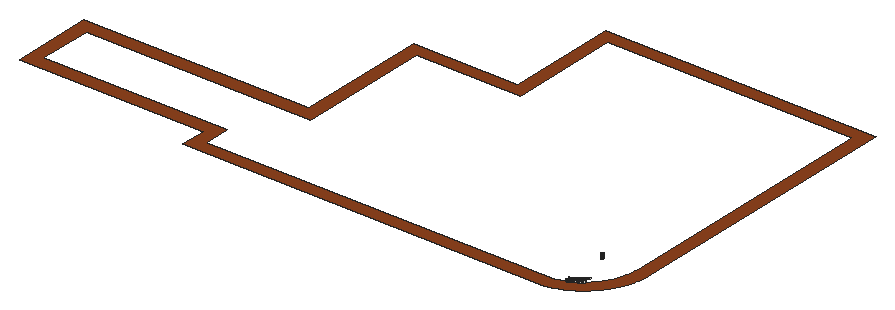
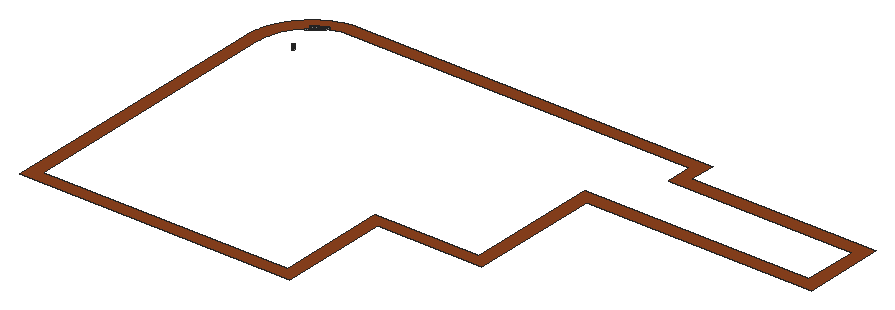
# SketchUp Ruby script. Lengths in inches.
U = 1.inch
M = Sketchup.active_model
def pt(a) = Geom::Point3d.new(a.map { |v| v * U })
def face(e, loops, mat)
  f = e.add_face(loops[0].map { |a| pt(a) })
  loops[1..].each { |l| e.add_face(l.map { |a| pt(a) }).erase! }
  f.material = f.back_material = mat if mat
  f
end
# faces: each face lists its corners as indices into pts; further lists are holes
def faces(e, pts, list, mat = nil) = list.each { |f| face(e, (f[0].is_a?(Array) ? f : [f]).map { |l| l.map { |i| pts[i] } }, mat) }
# xy, xz, yz: faces in a plane at the given z, y or x. An outline is a flat list of corners, or four numbers for a rectangle; further outlines are holes
def ring(l) = l.size == 4 ? [[l[0], l[1]], [l[2], l[1]], [l[2], l[3]], [l[0], l[3]]] : l.each_slice(2).to_a
def flat(e, list, mat, &to3) = list.each { |f| face(e, (f[0].is_a?(Array) ? f : [f]).map { |l| ring(l).map { |u, v| to3.(u, v) } }, mat) }
def xy(e, z, list, mat = nil) = flat(e, list, mat) { |x, y| [x, y, z] }
def xz(e, y, list, mat = nil) = flat(e, list, mat) { |x, z| [x, y, z] }
def yz(e, x, list, mat = nil) = flat(e, list, mat) { |y, z| [x, y, z] }
def lines(e, pts, list) = list.each { |a, b| e.add_line(pt(pts[a]), pt(pts[b])) }
# prism: a flat outline (further loops are holes) pulled along v
def prism(e, loops, v, mat = nil)
  f = face(e, loops, mat); d = Geom::Vector3d.new(v.map { |x| x * U })
  f.pushpull(f.normal.samedirection?(d) ? d.length : -d.length)
end
def box(e, o, s, mat = nil) = prism(e, [[o, [o[0] + s[0], o[1], o[2]], [o[0] + s[0], o[1] + s[1], o[2]], [o[0], o[1] + s[1], o[2]]]], [0, 0, s[2]], mat)
def at(x, y, z, deg = 0) = Geom::Transformation.translation(pt([x, y, z])) * Geom::Transformation.rotation(ORIGIN, Z_AXIS, deg.degrees)
def axes(o, x, y, z) = Geom::Transformation.new([*x, 0, *y, 0, *z, 0, *pt(o).to_a, 1])
def part(name) = M.definitions.add(name)
# library, detail: a bought-in or finely detailed component or shape, given as its bounding box
def library(name, o, s) = part(name).tap { |d| box(d.entities, o, s) }
def detail(e, o, s) = box(e.add_group.entities, o, s)
def put(e, d, t, mat = nil) = e.add_instance(d, t).tap { |i| i.material = mat if mat }
def group(e, t, mat = nil) = e.add_group.tap { |g| g.transformation = t; g.material = mat if mat }.entities
root = M.entities
M.materials.add("[Wood Fence]").color = [142, 67, 30]
xy(root,107.5,[[[126.5,152,126.5,166,26,166,26,210,149,210,149,282,206,282,206,342,354,342,354,186.72,353.99,186.41,353.98,186.09,353.96,185.77,353.95,185.45,353.93,185.13,353.9,184.8125,353.88,184.5,353.79,183.54,353.75,183.23,353.67,182.59,353.625,182.28,353.58,181.96,353.53,181.65,353.47,181.33,353.42,181.02,353.36,180.71,353.3,180.39,352.95,178.84,352.79,178.22,352.7,177.91,352.62,177.6,352.53,177.3,352.4375,176.99,352.34,176.6875,352.25,176.38,352.15,176.08,352.04,175.78,351.9375,175.48,351.83,175.18,351.61,174.58,351.49,174.28,351.37,173.99,351.25,173.69,351.13,173.4,351,173.11,350.875,172.8125,350.74,172.52,350.61,172.23,350.47,171.95,350.19,171.37,350.05,171.09,349.9,170.81,349.75,170.52,349.45,169.96,349.29,169.6875,349.13,169.41,348.97,169.13,348.8,168.86,348.64,168.59,348.3,168.05,348.125,167.78,347.95,167.52,347.77,167.25,347.41,166.73,346.84,165.95,346.65,165.7,346.46,165.44,346.26,165.19,346.0625,164.94,345.86,164.7,345.66,164.45,345.45,164.21,345.25,163.96,345.04,163.72,344.83,163.49,344.61,163.25,344.4,163.01,343.74,162.32,343.29,161.87,342.6,161.21,342.36,160.99,342.125,160.77,341.89,160.5625,341.65,160.35,341.41,160.14,341.16,159.9375,340.92,159.73,340.17,159.13,339.92,158.9375,339.67,158.75,339.41,158.55,339.15,158.37,338.9,158.18,338.64,158,338.375,157.8125,338.11,157.63,337.84,157.46,337.58,157.28,336.77,156.77,336.49,156.61,336.22,156.45,335.94,156.29,335.67,156.13,335.39,155.97,334.83,155.67,334.54,155.52,334.26,155.38,333.98,155.23,333.6875,155.09,333.4,154.96,333.11,154.82,332.82,154.6875,332.53,154.56,332.24,154.43,331.95,154.31,331.65,154.18,331.36,154.06,331.06,153.95,330.76,153.83,330.16,153.61,329.86,153.51,329.56,153.4,329.26,153.3,328.95,153.2,328.65,153.11,328.35,153.01,328.04,152.92,327.73,152.84,327.43,152.75,326.5,152.51,326.1875,152.44,325.88,152.37,325.57,152.3,325.25,152.23,324.63,152.11,324.3125,152.05,324,152],[133.5,159,323.38,159,323.59,159.04,323.84,159.09,324.1,159.14,325.1,159.38,325.34,159.44,326.09,159.65,326.33,159.72,326.58,159.79,326.83,159.87,327.07,159.95,327.3125,160.03,327.56,160.12,327.8,160.2,328.52,160.47,328.76,160.57,329,160.66,329.23,160.76,329.71,160.96,329.94,161.07,330.17,161.17,330.41,161.28,330.64,161.39,330.87,161.51,331.1,161.62,331.56,161.86,331.78,161.98,332.01,162.1,332.23,162.23,332.46,162.35,332.9,162.61,333.12,162.75,333.34,162.88,333.55,163.02,333.99,163.3,334.2,163.44,334.41,163.59,334.625,163.73,334.83,163.88,335.25,164.18,335.46,164.34,335.66,164.49,335.86,164.65,336.0625,164.81,336.26,164.97,336.46,165.13,336.66,165.3,336.86,165.46,337.24,165.8,337.4375,165.97,337.625,166.14,337.8125,166.32,338,166.49,338.1875,166.67,338.37,166.85,338.55,167.03,338.73,167.22,338.91,167.4,339.09,167.59,339.26,167.77,339.4375,167.96,339.61,168.15,339.78,168.35,339.95,168.54,340.12,168.74,340.28,168.93,340.45,169.13,340.93,169.73,341.08,169.9375,341.24,170.14,341.84,170.98,341.98,171.1875,342.125,171.4,342.27,171.61,342.55,172.05,342.68,172.27,342.82,172.48,342.95,172.7,343.08,172.93,343.21,173.15,343.33,173.37,343.46,173.6,343.58,173.82,343.82,174.28,343.93,174.51,344.05,174.74,344.27,175.2,344.375,175.43,344.48,175.67,344.59,175.9,344.6875,176.14,344.79,176.375,344.88,176.61,344.98,176.85,345.25,177.57,345.34,177.82,345.42,178.06,345.51,178.3,345.59,178.55,345.67,178.79,345.74,179.04,345.82,179.28,345.96,179.78,346.02,180.02,346.09,180.27,346.33,181.27,346.43,181.77,346.48,182.03,346.58,182.53,346.62,182.79,346.7,183.29,346.73,183.55,346.77,183.8,346.8,184.06,346.83,184.3125,346.86,184.57,346.88,184.82,346.92,185.34,346.94,185.59,346.96,185.85,346.97,186.1,346.99,186.62,347,186.875,347,335,213,335,213,275,156,275,156,203,33,203,33,173,133.5,173]]],"[Wood Fence]")
p = [[329.47,160.86,107.5],[329.23,160.76,107.5],[329.23,160.76,108.5],[329.47,160.86,108.5],[329.71,160.96,107.5],[329.71,160.96,108.5],
  [329.94,161.07,107.5],[329.94,161.07,108.5],[330.17,161.17,107.5],[330.17,161.17,108.5],[330.41,161.28,107.5],[330.41,161.28,108.5],
  [330.64,161.39,107.5],[330.64,161.39,108.5],[330.87,161.51,107.5],[330.87,161.51,108.5],[331.1,161.62,107.5],[331.1,161.62,108.5],
  [331.33,161.74,107.5],[331.33,161.74,108.5],[331.56,161.86,107.5],[331.56,161.86,108.5],[331.78,161.98,107.5],[331.78,161.98,108.5],
  [332.01,162.1,107.5],[332.01,162.1,108.5],[332.23,162.23,107.5],[332.23,162.23,108.5],[332.46,162.35,107.5],[332.46,162.35,108.5],
  [332.68,162.48,107.5],[332.68,162.48,108.5],[332.9,162.61,107.5],[332.9,162.61,108.5],[333.12,162.75,107.5],[333.12,162.75,108.5],
  [333.34,162.88,107.5],[333.34,162.88,108.5],[333.55,163.02,107.5],[333.55,163.02,108.5],[333.77,163.16,107.5],[333.77,163.16,108.5],
  [333.99,163.3,107.5],[333.99,163.3,108.5],[334.2,163.44,107.5],[334.2,163.44,108.5],[334.41,163.59,107.5],[334.41,163.59,108.5],
  [334.625,163.73,107.5],[334.625,163.73,108.5],[334.83,163.88,107.5],[334.83,163.88,108.5],[335.04,164.03,107.5],[335.04,164.03,108.5],
  [335.25,164.18,107.5],[335.25,164.18,108.5],[335.46,164.34,107.5],[335.46,164.34,108.5],[335.66,164.49,107.5],[335.66,164.49,108.5],
  [335.86,164.65,107.5],[335.86,164.65,108.5],[336.0625,164.81,107.5],[336.0625,164.81,108.5],[336.26,164.97,107.5],[336.26,164.97,108.5],
  [336.46,165.13,107.5],[336.46,165.13,108.5],[336.66,165.3,107.5],[336.66,165.3,108.5],[329.34,162.99,108],[329.55,163.09,108],
  [329.55,163.09,108.5],[329.34,162.99,108.5],[329.77,163.19,108],[329.77,163.19,108.5],[329.98,163.3,108],[329.98,163.3,108.5],
  [330.2,163.41,108],[330.2,163.41,108.5],[330.41,163.52,108],[330.41,163.52,108.5],[330.62,163.625,108],[330.62,163.625,108.5],
  [330.83,163.74,108],[330.83,163.74,108.5],[331.04,163.85,108],[331.04,163.85,108.5],[331.25,163.97,108],[331.25,163.97,108.5],
  [331.46,164.09,108],[331.46,164.09,108.5],[331.67,164.21,108],[331.67,164.21,108.5],[331.87,164.33,108],[331.87,164.33,108.5],
  [332.08,164.45,108],[332.08,164.45,108.5],[332.28,164.58,108],[332.28,164.58,108.5],[332.48,164.71,108],[332.48,164.71,108.5],
  [332.68,164.84,108],[332.68,164.84,108.5],[332.88,164.97,108],[332.88,164.97,108.5],[333.08,165.1,108],[333.08,165.1,108.5],
  [333.28,165.23,108],[333.28,165.23,108.5],[333.48,165.37,108],[333.48,165.37,108.5],[333.67,165.51,108],[333.67,165.51,108.5],
  [333.87,165.65,108],[333.87,165.65,108.5],[334.06,165.79,108],[334.06,165.79,108.5],[334.25,165.93,108],[334.25,165.93,108.5],
  [334.44,166.08,108],[334.44,166.08,108.5],[334.63,166.22,108],[334.63,166.22,108.5],[334.82,166.37,108],[334.82,166.37,108.5],
  [335.01,166.52,108],[335.01,166.52,108.5],[335.19,166.67,108],[335.19,166.67,108.5],[335.375,166.83,108],[335.375,166.83,108.5],
  [335.56,166.98,108],[335.56,166.98,108.5],[335.74,167.14,108],[335.74,167.14,108.5],[335.92,167.3,108],[335.92,167.3,108.5],
  [336.1,167.46,108],[336.1,167.46,108.5],[336.27,167.62,108],[336.27,167.62,108.5],[336.45,167.78,108],[336.45,167.78,108.5],
  [336.62,167.94,108],[336.62,167.94,108.5],[336.79,168.11,108],[336.79,168.11,108.5],[329.3125,185.02,108],[329.24,185.01,108],
  [329.24,185.01,111],[329.3125,185.02,111],[329.39,185.03,108],[329.39,185.03,111],[329.47,185.04,108],[329.47,185.04,111],
  [329.55,185.05,108],[329.55,185.05,111],[329.625,185.07,108],[329.625,185.07,111],[329.7,185.08,108],[329.7,185.08,111],
  [329.78,185.1,108],[329.78,185.1,111],[329.85,185.125,108],[329.85,185.125,111],[329.93,185.15,108],[329.93,185.15,111],
  [330,185.17,108],[330,185.17,111],[330.08,185.2,108],[330.08,185.2,111],[330.15,185.23,108],[330.15,185.23,111],
  [330.22,185.26,108],[330.22,185.26,111]]
faces(root,p,[[0,1,2,3],[4,0,3,5],[6,4,5,7],[8,6,7,9],[10,8,9,11],[12,10,11,13],[14,12,13,15],[16,14,15,17],
  [18,16,17,19],[20,18,19,21],[22,20,21,23],[24,22,23,25],[26,24,25,27],[28,26,27,29],[30,28,29,31],[32,30,31,33],
  [34,32,33,35],[36,34,35,37],[38,36,37,39],[40,38,39,41],[42,40,41,43],[44,42,43,45],[46,44,45,47],[48,46,47,49],
  [50,48,49,51],[52,50,51,53],[54,52,53,55],[56,54,55,57],[58,56,57,59],[60,58,59,61],[62,60,61,63],[64,62,63,65],
  [66,64,65,67],[68,66,67,69],[70,71,72,73],[71,74,75,72],[74,76,77,75],[76,78,79,77],[78,80,81,79],[80,82,83,81],
  [82,84,85,83],[84,86,87,85],[86,88,89,87],[88,90,91,89],[90,92,93,91],[92,94,95,93],[94,96,97,95],[96,98,99,97],
  [98,100,101,99],[100,102,103,101],[102,104,105,103],[104,106,107,105],[106,108,109,107],[108,110,111,109],[110,112,113,111],[112,114,115,113],
  [114,116,117,115],[116,118,119,117],[118,120,121,119],[120,122,123,121],[122,124,125,123],[124,126,127,125],[126,128,129,127],[128,130,131,129],
  [130,132,133,131],[132,134,135,133],[134,136,137,135],[136,138,139,137],[138,140,141,139],[140,142,143,141],[142,144,145,143],[144,146,147,145],
  [148,149,150,151],[152,148,151,153],[154,152,153,155],[156,154,155,157],[158,156,157,159],[160,158,159,161],[162,160,161,163],[164,162,163,165],
  [166,164,165,167],[168,166,167,169],[170,168,169,171],[172,170,171,173],[174,172,173,175]])
